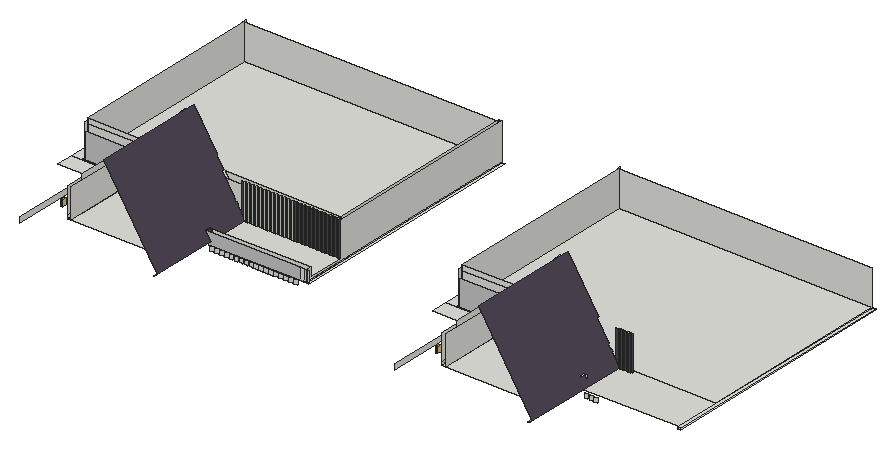
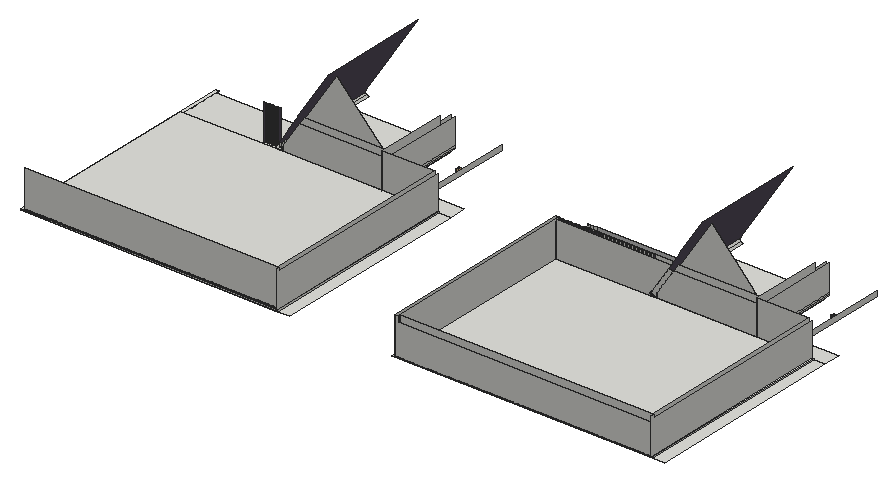
# SketchUp Ruby script. Lengths in inches.
U = 1.inch
M = Sketchup.active_model
def pt(a) = Geom::Point3d.new(a.map { |v| v * U })
def face(e, loops, mat)
  f = e.add_face(loops[0].map { |a| pt(a) })
  loops[1..].each { |l| e.add_face(l.map { |a| pt(a) }).erase! }
  f.material = f.back_material = mat if mat
  f
end
# faces: each face lists its corners as indices into pts; further lists are holes
def faces(e, pts, list, mat = nil) = list.each { |f| face(e, (f[0].is_a?(Array) ? f : [f]).map { |l| l.map { |i| pts[i] } }, mat) }
# xy, xz, yz: faces in a plane at the given z, y or x. An outline is a flat list of corners, or four numbers for a rectangle; further outlines are holes
def ring(l) = l.size == 4 ? [[l[0], l[1]], [l[2], l[1]], [l[2], l[3]], [l[0], l[3]]] : l.each_slice(2).to_a
def flat(e, list, mat, &to3) = list.each { |f| face(e, (f[0].is_a?(Array) ? f : [f]).map { |l| ring(l).map { |u, v| to3.(u, v) } }, mat) }
def xy(e, z, list, mat = nil) = flat(e, list, mat) { |x, y| [x, y, z] }
def xz(e, y, list, mat = nil) = flat(e, list, mat) { |x, z| [x, y, z] }
def yz(e, x, list, mat = nil) = flat(e, list, mat) { |y, z| [x, y, z] }
def lines(e, pts, list) = list.each { |a, b| e.add_line(pt(pts[a]), pt(pts[b])) }
# prism: a flat outline (further loops are holes) pulled along v
def prism(e, loops, v, mat = nil)
  f = face(e, loops, mat); d = Geom::Vector3d.new(v.map { |x| x * U })
  f.pushpull(f.normal.samedirection?(d) ? d.length : -d.length)
end
def box(e, o, s, mat = nil) = prism(e, [[o, [o[0] + s[0], o[1], o[2]], [o[0] + s[0], o[1] + s[1], o[2]], [o[0], o[1] + s[1], o[2]]]], [0, 0, s[2]], mat)
def at(x, y, z, deg = 0) = Geom::Transformation.translation(pt([x, y, z])) * Geom::Transformation.rotation(ORIGIN, Z_AXIS, deg.degrees)
def axes(o, x, y, z) = Geom::Transformation.new([*x, 0, *y, 0, *z, 0, *pt(o).to_a, 1])
def part(name) = M.definitions.add(name)
# library, detail: a bought-in or finely detailed component or shape, given as its bounding box
def library(name, o, s) = part(name).tap { |d| box(d.entities, o, s) }
def detail(e, o, s) = box(e.add_group.entities, o, s)
def put(e, d, t, mat = nil) = e.add_instance(d, t).tap { |i| i.material = mat if mat }
def group(e, t, mat = nil) = e.add_group.tap { |g| g.transformation = t; g.material = mat if mat }.entities
root = M.entities
M.materials.add("[Color M02]").color = [198, 198, 198]
M.materials.add("[Color M06]").color = [79, 71, 84]
M.materials.add("[Color M07]").color = [58, 58, 58]
c1 = library("Group\#13",[0,0,0],[3.54,3.54,3.9375])
xy(root,240.47,[[463.64,567.01,468.02,591.8125],[463.64,591.8125,468.02,646.3125],[468.02,591.8125,478.78,646.3125],[1350.1,591.8125,1354.48,646.3125],[1354.48,591.8125,1365.24,646.3125]])
xy(root,251.0625,[[478.78,562.32,478.78,732.32,312.41,732.32,312.41,1195.68,910.57,1195.68,910.57,630.04,671.33,630.04,671.33,562.32],[1365.24,562.32,1365.24,732.32,1198.87,732.32,1198.87,1195.68,1797.03,1195.68,1797.03,630.04,1557.79,630.04,1557.79,562.32],[435.78,567.01,446.59,646.3125],[446.59,567.01,463.64,646.3125],[463.64,567.01,463.64,646.3125,446.59,646.3125,446.59,732.32,478.78,732.32,478.78,567.01],
  [1322.24,567.01,1333.06,646.3125],[1333.06,567.01,1350.1,646.3125],[1350.1,567.01,1350.1,646.3125,1333.06,646.3125,1333.06,732.32,1365.24,732.32,1365.24,567.01],[910.57,623.84,910.57,1195.68,312.41,1195.68,312.41,732.32,435.78,732.32,435.78,726.125,424.39,726.125,424.39,686.3125,363.02,686.3125,363.02,726.125,306.21,726.125,306.21,1201.875,916.77,1201.875,916.77,623.84],[916.77,623.84,923.77,1201.875],
  [1797.03,623.84,1797.03,1195.68,1198.87,1195.68,1198.87,732.32,1322.24,732.32,1322.24,726.125,1310.86,726.125,1310.86,686.3125,1249.48,686.3125,1249.48,726.125,1192.67,726.125,1192.67,1201.875,1803.23,1201.875,1803.23,623.84],[424.39,646.3125,435.78,726.125],[435.78,646.3125,446.59,732.32],[1310.86,646.3125,1322.24,726.125],[1322.24,646.3125,1333.06,732.32],
  [278.96,686.3125,363.02,726.125],[1165.42,686.3125,1249.48,726.125],[278.96,726.125,306.21,1201.875],[1165.42,726.125,1192.67,1201.875]])
xy(root,253.4375,[[429.58,541.0625,435.78,541.0625,435.78,732.32,312.41,732.32,312.41,1195.68,910.57,1195.68,910.57,623.84,916.77,623.84,916.77,1201.875,310.02,1201.875,310.02,726.125,363.02,726.125,363.02,686.3125,429.58,686.3125],[1316.04,541.0625,1322.24,541.0625,1322.24,732.32,1198.87,732.32,1198.87,1195.68,1797.03,1195.68,1797.03,623.84,1803.23,623.84,1803.23,1201.875,1196.48,1201.875,1196.48,726.125,1249.48,726.125,1249.48,686.3125,1316.04,686.3125],[306.21,726.125,310.02,1201.875],[1192.67,726.125,1196.48,1201.875]])
xy(root,257.0625,[[671.46,521.5625,677.53,726.125],[1557.92,521.5625,1563.99,726.125],[428,528.48,435.78,719.59],[435.78,528.48,436.5,719.59],[436.5,528.48,671.46,719.59],
  [1314.46,528.48,1322.24,719.59],[1322.24,528.48,1322.96,719.59],[1322.96,528.48,1557.92,719.59],[677.53,636.82,916.77,636.82,916.77,724.8125,910.69,724.8125,910.69,726.125,907.27,726.125,907.27,724.8125,901.19,724.8125,901.19,726.125,897.77,726.125,897.77,724.8125,891.69,724.8125,891.69,726.125,888.27,726.125,888.27,724.8125,882.19,724.8125,882.19,726.125,878.77,726.125,878.77,724.8125,872.69,724.8125,872.69,726.125,869.27,726.125,869.27,724.8125,863.19,724.8125,863.19,726.125,859.77,726.125,859.77,724.8125,853.69,724.8125,853.69,726.125,850.27,726.125,850.27,724.8125,844.19,724.8125,844.19,726.125,840.77,726.125,840.77,724.8125,834.69,724.8125,834.69,726.125,831.27,726.125,831.27,724.8125,825.19,724.8125,825.19,726.125,821.77,726.125,821.77,724.8125,815.69,724.8125,815.69,726.125,812.27,726.125,812.27,724.8125,806.19,724.8125,806.19,726.125,802.77,726.125,802.77,724.8125,796.69,724.8125,796.69,726.125,793.27,726.125,793.27,724.8125,787.19,724.8125,787.19,726.125,783.77,726.125,783.77,724.8125,777.69,724.8125,777.69,726.125,774.27,726.125,774.27,724.8125,768.19,724.8125,768.19,726.125,764.77,726.125,764.77,724.8125,758.69,724.8125,758.69,726.125,755.27,726.125,755.27,724.8125,749.19,724.8125,749.19,726.125,745.77,726.125,745.77,724.8125,739.69,724.8125,739.69,726.125,736.27,726.125,736.27,724.8125,730.19,724.8125,730.19,726.125,726.77,726.125,726.77,724.8125,720.69,724.8125,720.69,726.125,717.27,726.125,717.27,724.8125,711.19,724.8125,711.19,726.125,707.77,726.125,707.77,724.8125,701.69,724.8125,701.69,726.125,698.27,726.125,698.27,724.8125,692.19,724.8125,692.19,726.125,677.53,726.125],[429.58,719.59,435.78,726.125],
  [435.78,719.59,436.5,726.125],[436.5,719.59,671.46,726.125],[1316.04,719.59,1322.24,726.125],[1322.24,719.59,1322.96,726.125],[1322.96,719.59,1557.92,726.125],
  [692.19,724.8125,692.19,726.125,677.53,726.125,677.53,732.2,910.69,732.2,910.69,726.125,907.27,726.125,907.27,724.8125,901.19,724.8125,901.19,726.125,897.77,726.125,897.77,724.8125,891.69,724.8125,891.69,726.125,888.27,726.125,888.27,724.8125,882.19,724.8125,882.19,726.125,878.77,726.125,878.77,724.8125,872.69,724.8125,872.69,726.125,869.27,726.125,869.27,724.8125,863.19,724.8125,863.19,726.125,859.77,726.125,859.77,724.8125,853.69,724.8125,853.69,726.125,850.27,726.125,850.27,724.8125,844.19,724.8125,844.19,726.125,840.77,726.125,840.77,724.8125,834.69,724.8125,834.69,726.125,831.27,726.125,831.27,724.8125,825.19,724.8125,825.19,726.125,821.77,726.125,821.77,724.8125,815.69,724.8125,815.69,726.125,812.27,726.125,812.27,724.8125,806.19,724.8125,806.19,726.125,802.77,726.125,802.77,724.8125,796.69,724.8125,796.69,726.125,793.27,726.125,793.27,724.8125,787.19,724.8125,787.19,726.125,783.77,726.125,783.77,724.8125,777.69,724.8125,777.69,726.125,774.27,726.125,774.27,724.8125,768.19,724.8125,768.19,726.125,764.77,726.125,764.77,724.8125,758.69,724.8125,758.69,726.125,755.27,726.125,755.27,724.8125,749.19,724.8125,749.19,726.125,745.77,726.125,745.77,724.8125,739.69,724.8125,739.69,726.125,736.27,726.125,736.27,724.8125,730.19,724.8125,730.19,726.125,726.77,726.125,726.77,724.8125,720.69,724.8125,720.69,726.125,717.27,726.125,717.27,724.8125,711.19,724.8125,711.19,726.125,707.77,726.125,707.77,724.8125,701.69,724.8125,701.69,726.125,698.27,726.125,698.27,724.8125],[436.5,726.125,671.46,732.2],[671.46,726.125,677.53,732.2],[1322.96,726.125,1557.92,732.2],[1557.92,726.125,1563.99,732.2],
  [312.28,732.2,677.53,732.2,677.53,734.4375,910.69,734.4375,910.69,1195.8,312.28,1195.8],[677.53,732.2,910.69,734.4375],[1198.75,732.2,1563.99,732.2,1563.99,734.4375,1797.15,734.4375,1797.15,1195.8,1198.75,1195.8]])
xz(root,620.37,[[691.13,240.88,699.82,251.0625],[702.82,240.88,711.51,251.0625],[714.51,240.88,723.19,251.0625],[726.19,240.88,734.88,251.0625],[737.88,240.88,746.57,251.0625],
  [749.57,240.88,758.26,251.0625],[761.26,240.88,769.94,251.0625],[772.94,240.88,781.63,251.0625],[784.63,240.88,793.32,251.0625],[796.32,240.88,805.01,251.0625],
  [808.01,240.88,816.69,251.0625],[819.69,240.88,828.38,251.0625],[831.38,240.88,840.07,251.0625],[843.07,240.88,851.76,251.0625],[854.76,240.88,863.44,251.0625],
  [866.44,240.88,875.13,251.0625],[878.13,240.88,886.82,251.0625],[889.82,240.88,898.51,251.0625],[1577.59,240.88,1586.28,251.0625],[1589.28,240.88,1597.97,251.0625],
  [1600.97,240.88,1609.66,251.0625]])
xz(root,623.84,[[901.22,251.0625,910.57,278.1875],[910.57,251.0625,916.77,253.4375],[916.77,251.0625,923.77,253.4375],[910.57,253.4375,916.77,278.1875],[916.77,253.4375,923.77,278.1875]])
xz(root,623.84,[[686.84,251.0625,901.22,251.0625,901.22,278.1875,677.53,278.1875,677.53,257.0625,686.84,257.0625]],"[Color M02]")
xz(root,636.82,[[677.53,257.0625,683.25,278.1875],[683.25,257.0625,916.77,278.1875],[1563.99,257.0625,1569.71,278.1875]])
xz(root,686.3125,[[363.02,251.0625,429.58,253.4375],[1249.48,251.0625,1316.04,253.4375]])
xz(root,719.59,[[428,257.0625,429.58,258.95],[429.58,257.0625,429.58,263.89,428,263.89,428,326.08,436.5,326.08,436.5,257.0625],[436.5,257.0625,671.46,257.0625,671.46,266.53,553.56,450.4375,459.19,350.1875,449.72,340.125,436.5,326.08],[1314.46,257.0625,1316.04,258.95],[1316.04,257.0625,1316.04,263.89,1314.46,263.89,1314.46,326.08,1322.96,326.08,1322.96,257.0625],
  [1322.96,257.0625,1557.92,257.0625,1557.92,266.53,1440.02,450.4375,1345.65,350.1875,1336.18,340.125,1322.96,326.08],[428,258.95,429.58,263.89],[1314.46,258.95,1316.04,263.89]])
xz(root,724.8125,[[692.19,257.0625,698.27,340.125],[701.69,257.0625,707.77,340.125],[711.19,257.0625,717.27,340.125],[720.69,257.0625,726.77,340.125],[730.19,257.0625,736.27,340.125],
  [739.69,257.0625,745.77,340.125],[749.19,257.0625,755.27,340.125],[758.69,257.0625,764.77,340.125],[768.19,257.0625,774.27,340.125],[777.69,257.0625,783.77,340.125],
  [787.19,257.0625,793.27,340.125],[796.69,257.0625,802.77,340.125],[806.19,257.0625,812.27,340.125],[815.69,257.0625,821.77,340.125],[825.19,257.0625,831.27,340.125],
  [834.69,257.0625,840.77,340.125],[844.19,257.0625,850.27,340.125],[853.69,257.0625,859.77,340.125],[863.19,257.0625,869.27,340.125],[872.69,257.0625,878.77,340.125],
  [882.19,257.0625,888.27,340.125],[891.69,257.0625,897.77,340.125],[901.19,257.0625,907.27,340.125],[910.69,257.0625,916.77,340.125],[1578.65,257.0625,1584.73,340.125],
  [1588.15,257.0625,1594.23,340.125],[1597.65,257.0625,1603.73,340.125],[688.77,260.03,688.77,340.125,682.69,340.125,682.69,269.51,682.79,269.35,686.84,263.03],[1575.23,260.03,1575.23,340.125,1569.15,340.125,1569.15,269.51,1569.26,269.35,1573.31,263.03]],"[Color M06]")
xz(root,726.125,[[306.21,251.0625,363.02,253.4375],[424.39,251.0625,435.78,251.0625,435.78,257.0625,429.58,257.0625,429.58,258.95,424.39,258.95],[1192.67,251.0625,1249.48,253.4375],[1310.86,251.0625,1322.24,251.0625,1322.24,257.0625,1316.04,257.0625,1316.04,258.95,1310.86,258.95],[680.77,252.01,677.53,257.0625,683.25,257.0625,684.82,254.61],
  [1567.23,252.01,1563.99,257.0625,1569.71,257.0625,1571.28,254.61],[684.82,254.61,683.25,257.0625,688.65,257.0625],[1571.28,254.61,1569.71,257.0625,1575.11,257.0625],[436.5,257.0625,663.69,257.0625,663.69,278.65,624.28,340.125,436.5,340.125],[663.69,257.0625,669.77,257.0625,669.77,269.17,663.69,278.65],
  [669.77,257.0625,673.19,257.0625,673.19,263.83,671.46,266.53,669.77,269.17],[673.19,257.0625,677.53,257.0625,673.19,263.83],[677.53,257.0625,677.53,265.98,673.19,272.75,673.19,263.83],[677.53,257.0625,679.27,257.0625,679.27,258.18],[677.53,257.0625,679.27,258.18,679.27,263.27,677.53,265.98],
  [679.27,257.0625,682.69,257.0625,682.69,257.93,681.58,259.66,679.27,258.18],[682.69,257.0625,683.25,257.0625,682.69,257.93],[683.25,257.0625,688.65,257.0625,688.77,257.14,688.77,260.03,686.84,263.03,682.69,260.37,682.69,257.93],[688.65,257.0625,688.77,257.0625,688.77,257.14],[1322.96,257.0625,1550.15,257.0625,1550.15,278.65,1510.74,340.125,1322.96,340.125],
  [1550.15,257.0625,1556.23,257.0625,1556.23,269.17,1550.15,278.65],[1556.23,257.0625,1559.65,257.0625,1559.65,263.83,1557.92,266.53,1556.23,269.17],[1559.65,257.0625,1563.99,257.0625,1559.65,263.83],[1563.99,257.0625,1563.99,265.98,1559.65,272.75,1559.65,263.83],[1563.99,257.0625,1565.73,257.0625,1565.73,258.18],
  [1563.99,257.0625,1565.73,258.18,1565.73,263.27,1563.99,265.98],[1565.73,257.0625,1569.15,257.0625,1569.15,257.93,1568.05,259.66,1565.73,258.18],[1569.15,257.0625,1569.71,257.0625,1569.15,257.93],[1569.71,257.0625,1575.11,257.0625,1575.23,257.14,1575.23,260.03,1573.31,263.03,1569.15,260.37,1569.15,257.93],[1575.11,257.0625,1575.23,257.0625,1575.23,257.14],
  [688.77,257.14,690.08,257.98,688.77,260.03],[1575.23,257.14,1576.55,257.98,1575.23,260.03],[682.69,257.93,682.69,260.37,681.58,259.66],[1569.15,257.93,1569.15,260.37,1568.05,259.66],[679.27,258.18,681.58,259.66,679.27,263.27],
  [1565.73,258.18,1568.05,259.66,1565.73,263.27],[363.02,258.95,424.39,263.89],[424.39,258.95,429.58,263.89],[1249.48,258.95,1310.86,263.89],[1310.86,258.95,1316.04,263.89],
  [681.58,259.66,682.69,260.37,682.69,269.29,679.27,267.09,679.27,263.27],[1568.05,259.66,1569.15,260.37,1569.15,269.29,1565.73,267.09,1565.73,263.27],[682.69,260.37,686.84,263.03,682.79,269.35,682.69,269.29],[1569.15,260.37,1573.31,263.03,1569.26,269.35,1569.15,269.29],[679.27,263.27,679.27,267.09,677.53,265.98],
  [1565.73,263.27,1565.73,267.09,1563.99,265.98],[673.19,263.83,673.19,272.75,669.77,278.09,669.77,269.17,671.46,266.53],[1559.65,263.83,1559.65,272.75,1556.23,278.09,1556.23,269.17,1557.92,266.53],[424.39,263.89,429.58,315.25],[1310.86,263.89,1316.04,315.25]])
xz(root,726.125,[[310.02,253.4375,363.02,253.4375,363.02,263.89,424.39,263.89,424.39,315.25,310.02,315.25],[1196.48,253.4375,1249.48,253.4375,1249.48,263.89,1310.86,263.89,1310.86,315.25,1196.48,315.25]],"[Color M02]")
xz(root,726.125,[[688.77,257.0625,692.19,257.0625,692.19,340.125,688.77,340.125,688.77,260.03,690.08,257.98,688.77,257.14],[698.27,257.0625,701.69,340.125],[707.77,257.0625,711.19,340.125],[717.27,257.0625,720.69,340.125],[726.77,257.0625,730.19,340.125],
  [736.27,257.0625,739.69,340.125],[745.77,257.0625,749.19,340.125],[755.27,257.0625,758.69,340.125],[764.77,257.0625,768.19,340.125],[774.27,257.0625,777.69,340.125],
  [783.77,257.0625,787.19,340.125],[793.27,257.0625,796.69,340.125],[802.77,257.0625,806.19,340.125],[812.27,257.0625,815.69,340.125],[821.77,257.0625,825.19,340.125],
  [831.27,257.0625,834.69,340.125],[840.77,257.0625,844.19,340.125],[850.27,257.0625,853.69,340.125],[859.77,257.0625,863.19,340.125],[869.27,257.0625,872.69,340.125],
  [878.77,257.0625,882.19,340.125],[888.27,257.0625,891.69,340.125],[897.77,257.0625,901.19,340.125],[907.27,257.0625,910.69,340.125],[1575.23,257.0625,1578.65,257.0625,1578.65,340.125,1575.23,340.125,1575.23,260.03,1576.55,257.98,1575.23,257.14],
  [1584.73,257.0625,1588.15,340.125],[1594.23,257.0625,1597.65,340.125],[1603.73,257.0625,1607.15,340.125]],"[Color M06]")
xz(root,732.2,[[312.28,257.0625,436.5,328],[436.5,257.0625,436.5,326.08,438.31,328,632.05,328,671.46,266.53,671.46,257.0625],[671.46,257.0625,671.46,266.53,632.05,328,910.57,328,910.57,340.125,910.69,340.125,910.69,257.0625],[1198.75,257.0625,1322.96,328],[1322.96,257.0625,1322.96,326.08,1324.77,328,1518.52,328,1557.92,266.53,1557.92,257.0625]])
xz(root,732.32,[[312.41,251.0625,435.78,253.4375],[1198.87,251.0625,1322.24,253.4375],[312.41,253.4375,435.78,340.125],[1198.87,253.4375,1322.24,340.125]])
xz(root,734.4375,[[677.53,257.0625,681.58,259.66,686.84,263.03,682.79,269.35,677.53,277.56,637.42,340.125,910.69,340.125,910.69,257.0625]])
xz(root,1195.68,[[312.41,251.0625,910.57,253.4375],[1198.87,251.0625,1797.03,253.4375],[312.41,253.4375,910.57,340.125],[1198.87,253.4375,1797.03,340.125]])
xz(root,1201.875,[[306.21,251.0625,916.77,253.4375],[1192.67,251.0625,1803.23,253.4375],[310.02,253.4375,310.02,328,910.57,328,910.57,340.125,916.77,340.125,916.77,253.4375]])
yz(root,306.21,[[726.125,251.0625,1201.875,253.4375]])
yz(root,310.02,[[726.125,253.4375,726.125,333.125,1195.68,333.125,1195.68,340.125,1201.875,340.125,1201.875,253.4375]])
yz(root,312.41,[[732.32,251.0625,1195.68,253.4375],[732.32,253.4375,1195.68,340.125]])
yz(root,363.02,[[469.875,251.0625,469.875,263.89,726.125,263.89,726.125,253.4375,686.3125,253.4375,686.3125,251.0625],[686.3125,251.0625,726.125,253.4375]])
yz(root,428,[[528.48,257.0625,719.59,258.95],[528.48,258.95,719.59,263.89],[528.48,263.89,719.59,326.08]])
yz(root,429.58,[[719.59,257.0625,726.125,258.95],[719.59,258.95,726.125,263.89]])
yz(root,435.78,[[562.32,251.0625,726.125,253.4375],[726.125,251.0625,732.32,253.4375],[562.32,253.4375,726.125,257.0625],[726.125,253.4375,732.32,253.4375,732.32,340.125,562.32,340.125,562.32,257.0625,726.125,257.0625]])
yz(root,436.5,[[528.48,257.0625,719.59,326.08],[719.59,257.0625,726.125,326.08],[726.125,257.0625,732.2,326.08]])
yz(root,463.64,[[591.8125,240.47,646.3125,251.0625]],"[Color M07]")
yz(root,671.46,[[528.48,257.0625,719.59,266.53],[719.59,257.0625,732.2,266.53]])
yz(root,677.53,[[623.84,257.0625,636.82,278.1875]])
yz(root,688.77,[[724.8125,260.03,726.125,340.125]])
yz(root,692.19,[[724.8125,257.0625,726.125,340.125]])
yz(root,698.27,[[724.8125,257.0625,726.125,340.125]])
yz(root,701.69,[[724.8125,257.0625,726.125,340.125]])
yz(root,707.77,[[724.8125,257.0625,726.125,340.125]])
yz(root,711.19,[[724.8125,257.0625,726.125,340.125]])
yz(root,717.27,[[724.8125,257.0625,726.125,340.125]])
yz(root,720.69,[[724.8125,257.0625,726.125,340.125]])
yz(root,726.77,[[724.8125,257.0625,726.125,340.125]])
yz(root,730.19,[[724.8125,257.0625,726.125,340.125]])
yz(root,736.27,[[724.8125,257.0625,726.125,340.125]])
yz(root,739.69,[[724.8125,257.0625,726.125,340.125]])
yz(root,745.77,[[724.8125,257.0625,726.125,340.125]])
yz(root,749.19,[[724.8125,257.0625,726.125,340.125]])
yz(root,755.27,[[724.8125,257.0625,726.125,340.125]])
yz(root,758.69,[[724.8125,257.0625,726.125,340.125]])
yz(root,764.77,[[724.8125,257.0625,726.125,340.125]])
yz(root,768.19,[[724.8125,257.0625,726.125,340.125]])
yz(root,774.27,[[724.8125,257.0625,726.125,340.125]])
yz(root,777.69,[[724.8125,257.0625,726.125,340.125]])
yz(root,783.77,[[724.8125,257.0625,726.125,340.125]])
yz(root,787.19,[[724.8125,257.0625,726.125,340.125]])
yz(root,793.27,[[724.8125,257.0625,726.125,340.125]])
yz(root,796.69,[[724.8125,257.0625,726.125,340.125]])
yz(root,802.77,[[724.8125,257.0625,726.125,340.125]])
yz(root,806.19,[[724.8125,257.0625,726.125,340.125]])
yz(root,812.27,[[724.8125,257.0625,726.125,340.125]])
yz(root,815.69,[[724.8125,257.0625,726.125,340.125]])
yz(root,821.77,[[724.8125,257.0625,726.125,340.125]])
yz(root,825.19,[[724.8125,257.0625,726.125,340.125]])
yz(root,831.27,[[724.8125,257.0625,726.125,340.125]])
yz(root,834.69,[[724.8125,257.0625,726.125,340.125]])
yz(root,840.77,[[724.8125,257.0625,726.125,340.125]])
yz(root,844.19,[[724.8125,257.0625,726.125,340.125]])
yz(root,850.27,[[724.8125,257.0625,726.125,340.125]])
yz(root,853.69,[[724.8125,257.0625,726.125,340.125]])
yz(root,859.77,[[724.8125,257.0625,726.125,340.125]])
yz(root,863.19,[[724.8125,257.0625,726.125,340.125]])
yz(root,869.27,[[724.8125,257.0625,726.125,340.125]])
yz(root,872.69,[[724.8125,257.0625,726.125,340.125]])
yz(root,878.77,[[724.8125,257.0625,726.125,340.125]])
yz(root,882.19,[[724.8125,257.0625,726.125,340.125]])
yz(root,888.27,[[724.8125,257.0625,726.125,340.125]])
yz(root,891.69,[[724.8125,257.0625,726.125,340.125]])
yz(root,897.77,[[724.8125,257.0625,726.125,340.125]])
yz(root,901.19,[[724.8125,257.0625,726.125,340.125]])
yz(root,907.27,[[724.8125,257.0625,726.125,340.125]])
yz(root,910.57,[[623.84,251.0625,630.04,253.4375],[630.04,251.0625,1195.68,253.4375]])
yz(root,910.69,[[724.8125,257.0625,726.125,340.125],[726.125,257.0625,732.2,340.125],[732.2,257.0625,734.4375,340.125],[734.4375,257.0625,1195.8,340.125]])
yz(root,916.77,[[623.84,251.0625,1201.875,253.4375],[623.84,253.4375,1201.875,253.4375,1201.875,340.125,724.8125,340.125,724.8125,257.0625,636.82,257.0625,636.82,278.1875,623.84,278.1875]])
yz(root,1192.67,[[726.125,251.0625,1201.875,253.4375]])
yz(root,1196.48,[[726.125,253.4375,726.125,333.125,1195.68,333.125,1195.68,340.125,1201.875,340.125,1201.875,253.4375]])
yz(root,1198.87,[[732.32,251.0625,1195.68,253.4375],[732.32,253.4375,1195.68,340.125]])
yz(root,1249.48,[[469.875,251.0625,469.875,263.89,726.125,263.89,726.125,253.4375,686.3125,253.4375,686.3125,251.0625],[686.3125,251.0625,726.125,253.4375]])
yz(root,1314.46,[[528.48,257.0625,719.59,258.95],[528.48,258.95,719.59,263.89],[528.48,263.89,719.59,326.08]])
yz(root,1316.04,[[719.59,257.0625,726.125,258.95],[719.59,258.95,726.125,263.89]])
yz(root,1322.24,[[562.32,251.0625,726.125,253.4375],[726.125,251.0625,732.32,253.4375],[562.32,253.4375,726.125,257.0625],[726.125,253.4375,732.32,253.4375,732.32,340.125,562.32,340.125,562.32,257.0625,726.125,257.0625]])
yz(root,1322.96,[[528.48,257.0625,719.59,326.08],[719.59,257.0625,726.125,326.08],[726.125,257.0625,732.2,326.08]])
yz(root,1350.1,[[591.8125,240.47,646.3125,251.0625]],"[Color M07]")
yz(root,1557.92,[[528.48,257.0625,719.59,266.53],[719.59,257.0625,732.2,266.53]])
yz(root,1563.99,[[623.84,257.0625,636.82,278.1875]])
yz(root,1575.23,[[724.8125,260.03,726.125,340.125]])
yz(root,1578.65,[[724.8125,257.0625,726.125,340.125]])
yz(root,1584.73,[[724.8125,257.0625,726.125,340.125]])
yz(root,1588.15,[[724.8125,257.0625,726.125,340.125]])
yz(root,1594.23,[[724.8125,257.0625,726.125,340.125]])
yz(root,1597.65,[[724.8125,257.0625,726.125,340.125]])
yz(root,1603.73,[[724.8125,257.0625,726.125,340.125]])
p = [[680.77,719.59,252.01],[680.77,726.125,252.01],[684.82,726.125,254.61],[684.82,467.1875,254.61],[680.77,467.1875,252.01],[680.77,521.5625,252.01],
  [680.77,528.48,252.01],[680.77,623.84,252.01],[680.77,636.82,252.01],[1567.23,719.59,252.01],[1567.23,726.125,252.01],[1571.28,726.125,254.61],
  [1571.28,467.1875,254.61],[1567.23,467.1875,252.01],[1567.23,521.5625,252.01],[1567.23,528.48,252.01],[1567.23,623.84,252.01],[1567.23,636.82,252.01],
  [677.53,623.84,257.0625],[677.53,636.82,257.0625],[1563.99,623.84,257.0625],[1563.99,636.82,257.0625],[677.53,719.59,257.0625],[1563.99,719.59,257.0625],
  [677.53,726.125,257.0625],[1563.99,726.125,257.0625],[688.65,726.125,257.0625],[688.77,726.125,257.14],[690.08,726.125,257.98],[690.08,467.1875,257.98],
  [1575.11,726.125,257.0625],[1575.23,726.125,257.14],[1576.55,726.125,257.98],[1576.55,467.1875,257.98],[671.46,528.48,266.53],[671.46,719.59,266.53],
  [677.53,528.48,257.0625],[1557.92,528.48,266.53],[1557.92,719.59,266.53],[1563.99,528.48,257.0625],[671.46,726.125,266.53],[673.19,726.125,263.83],
  [1557.92,726.125,266.53],[1559.65,726.125,263.83],[679.27,726.125,258.18],[681.58,726.125,259.66],[681.58,734.4375,259.66],[677.53,734.4375,257.0625],
  [677.53,732.2,257.0625],[1565.73,726.125,258.18],[1568.05,726.125,259.66],[1568.05,734.4375,259.66],[1563.99,734.4375,257.0625],[1563.99,732.2,257.0625],
  [562.87,726.125,456.41],[562.87,467.1875,456.41],[686.29,467.1875,263.89],[686.84,467.1875,263.03],[688.77,726.125,260.03],[688.77,724.8125,260.03],
  [686.84,724.8125,263.03],[682.79,724.8125,269.35],[682.69,724.8125,269.51],[682.69,726.125,269.51],[679.27,726.125,274.85],[679.27,724.8125,274.85],
  [677.53,724.8125,277.56],[673.19,724.8125,284.33],[673.19,726.125,284.33],[669.77,726.125,289.67],[669.77,724.8125,289.67],[663.69,724.8125,299.15],
  [663.69,726.125,299.15],[637.42,726.125,340.125],[635.26,726.125,343.5],[635.26,732.2,343.5],[630.97,732.2,350.1875],[619.35,732.2,368.3125],
  [617.68,732.2,370.91],[562.87,732.2,456.41],[1449.33,726.125,456.41],[1449.33,467.1875,456.41],[1572.76,467.1875,263.89],[1573.31,467.1875,263.03],
  [1575.23,726.125,260.03],[1575.23,724.8125,260.03],[1573.31,724.8125,263.03],[1569.26,724.8125,269.35],[1569.15,724.8125,269.51],[1569.15,726.125,269.51],
  [1565.73,726.125,274.85],[1565.73,724.8125,274.85],[1563.99,724.8125,277.56],[1559.65,724.8125,284.33],[1559.65,726.125,284.33],[1556.23,726.125,289.67],
  [1556.23,724.8125,289.67],[1550.15,724.8125,299.15],[1550.15,726.125,299.15],[1523.88,726.125,340.125],[1521.72,726.125,343.5],[1521.72,732.2,343.5],
  [1517.43,732.2,350.1875],[1505.8125,732.2,368.3125],[1504.15,732.2,370.91],[1449.33,732.2,456.41],[682.69,726.125,260.37],[686.84,726.125,263.03],
  [686.84,734.4375,263.03],[1569.15,726.125,260.37],[1573.31,726.125,263.03],[1573.31,734.4375,263.03],[682.79,726.125,269.35],[1569.26,726.125,269.35],
  [682.79,734.4375,269.35],[1569.26,734.4375,269.35],[1563.71,636.82,257.0625],[1332.23,646.3125,240.47],[1332.23,686.3125,240.47],[445.77,646.3125,240.47],
  [445.77,686.3125,240.47],[677.25,636.82,257.0625]]
faces(root,p,[[0,1,2,3,4,5,6,7,8],[9,10,11,12,13,14,15,16,17],[18,19,8,7],[20,21,17,16],[19,22,0,8],[21,23,9,17],[22,24,1,0],[23,25,10,9],
  [3,2,26,27,28,29],[12,11,30,31,32,33],[34,35,22,19,18,36],[37,38,23,21,20,39],[22,35,40,41,24],[23,38,42,43,25],[24,44,45,46,47,48],[25,49,50,51,52,53],
  [45,106,107,108,46],[50,109,110,111,51],[58,107,60,59],[84,110,86,85],[107,112,61,60],[110,113,87,86],[107,112,114,108],[110,113,115,111]])
faces(root,p,[[54,55,56,57,29,28,58,59,60,61,62,63,64,65,66,67,68,69,70,71,72,73,74,75,76,77,78,79],[80,81,82,83,33,32,84,85,86,87,88,89,90,91,92,93,94,95,96,97,98,99,100,101,102,103,104,105]],"[Color M06]")
lines(root,p,[[21,116],[117,118],[119,120],[19,121]])
put(root,c1,axes([378.57,577,258.17],[-1.5535,0,0],[0,2.39,0],[0,0,-3.63878]))
put(root,c1,axes([1265.03,577,258.17],[-1.5535,0,0],[0,2.39,0],[0,0,-3.63878]))
